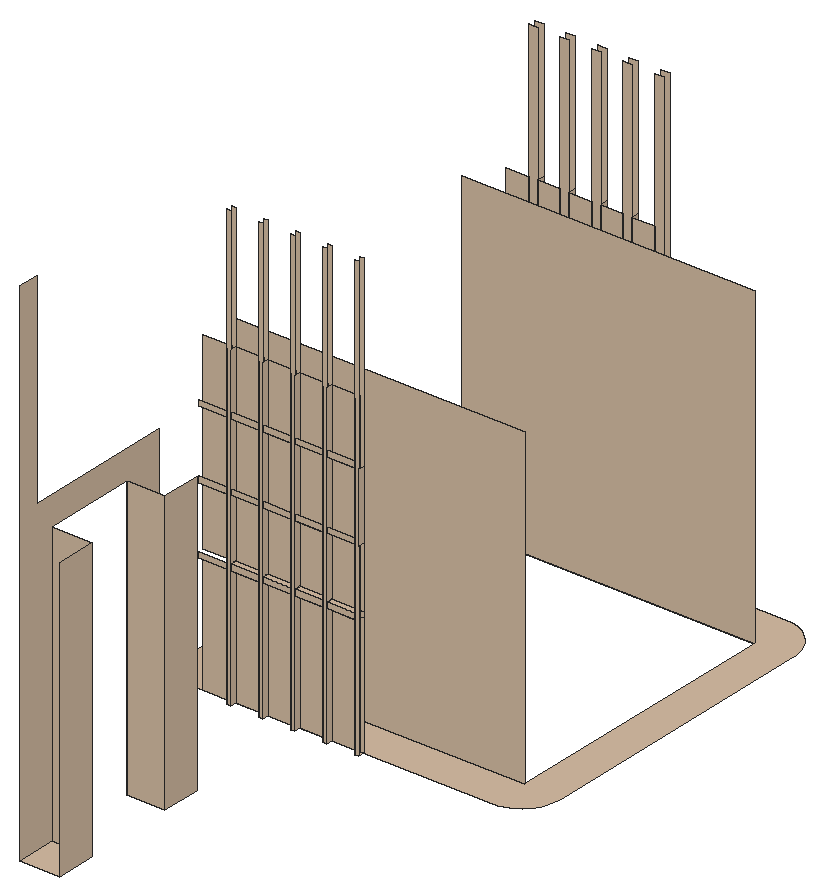
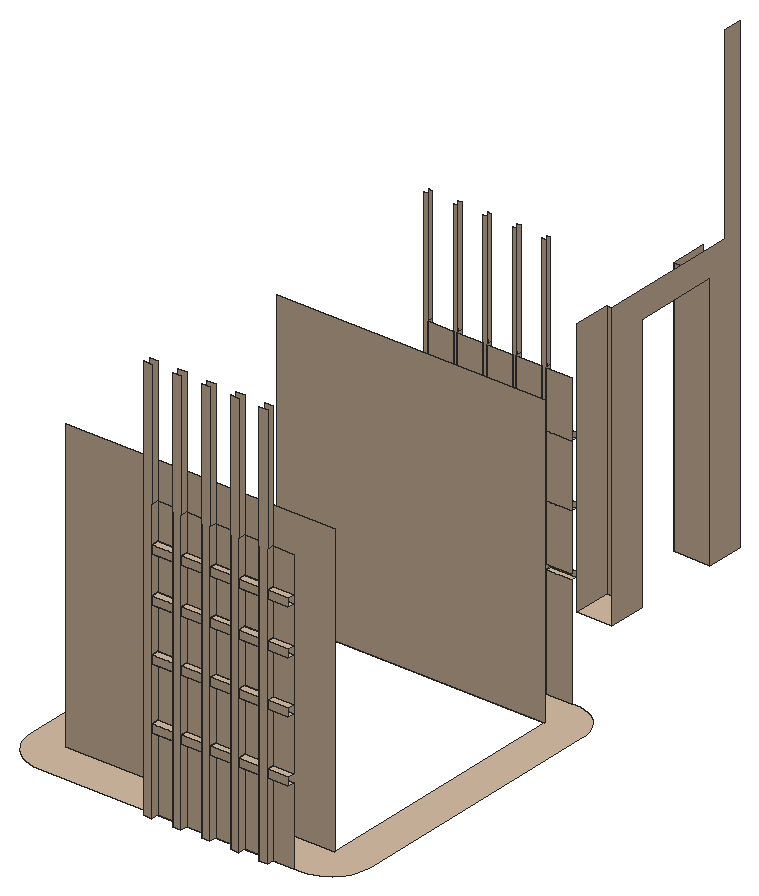
# SketchUp Ruby script. Lengths in inches.
U = 1.inch
M = Sketchup.active_model
def pt(a) = Geom::Point3d.new(a.map { |v| v * U })
def face(e, loops, mat)
  f = e.add_face(loops[0].map { |a| pt(a) })
  loops[1..].each { |l| e.add_face(l.map { |a| pt(a) }).erase! }
  f.material = f.back_material = mat if mat
  f
end
# faces: each face lists its corners as indices into pts; further lists are holes
def faces(e, pts, list, mat = nil) = list.each { |f| face(e, (f[0].is_a?(Array) ? f : [f]).map { |l| l.map { |i| pts[i] } }, mat) }
# xy, xz, yz: faces in a plane at the given z, y or x. An outline is a flat list of corners, or four numbers for a rectangle; further outlines are holes
def ring(l) = l.size == 4 ? [[l[0], l[1]], [l[2], l[1]], [l[2], l[3]], [l[0], l[3]]] : l.each_slice(2).to_a
def flat(e, list, mat, &to3) = list.each { |f| face(e, (f[0].is_a?(Array) ? f : [f]).map { |l| ring(l).map { |u, v| to3.(u, v) } }, mat) }
def xy(e, z, list, mat = nil) = flat(e, list, mat) { |x, y| [x, y, z] }
def xz(e, y, list, mat = nil) = flat(e, list, mat) { |x, z| [x, y, z] }
def yz(e, x, list, mat = nil) = flat(e, list, mat) { |y, z| [x, y, z] }
def lines(e, pts, list) = list.each { |a, b| e.add_line(pt(pts[a]), pt(pts[b])) }
# prism: a flat outline (further loops are holes) pulled along v
def prism(e, loops, v, mat = nil)
  f = face(e, loops, mat); d = Geom::Vector3d.new(v.map { |x| x * U })
  f.pushpull(f.normal.samedirection?(d) ? d.length : -d.length)
end
def box(e, o, s, mat = nil) = prism(e, [[o, [o[0] + s[0], o[1], o[2]], [o[0] + s[0], o[1] + s[1], o[2]], [o[0], o[1] + s[1], o[2]]]], [0, 0, s[2]], mat)
def at(x, y, z, deg = 0) = Geom::Transformation.translation(pt([x, y, z])) * Geom::Transformation.rotation(ORIGIN, Z_AXIS, deg.degrees)
def axes(o, x, y, z) = Geom::Transformation.new([*x, 0, *y, 0, *z, 0, *pt(o).to_a, 1])
def part(name) = M.definitions.add(name)
# library, detail: a bought-in or finely detailed component or shape, given as its bounding box
def library(name, o, s) = part(name).tap { |d| box(d.entities, o, s) }
def detail(e, o, s) = box(e.add_group.entities, o, s)
def put(e, d, t, mat = nil) = e.add_instance(d, t).tap { |i| i.material = mat if mat }
def group(e, t, mat = nil) = e.add_group.tap { |g| g.transformation = t; g.material = mat if mat }.entities
root = M.entities
M.materials.add("[Formica Laminate Light]").color = [213, 189, 164]
xy(root,0,[[297.89,97.95,301.53,101.59],[297.89,110.07,301.35,113.72],[295.1875,124.79,295.55,125.33],[298.11,124.79,298.47,125.33],[301.04,124.79,301.4,125.33],
  [303.96,124.79,304.32,125.33],[306.88,124.79,307.24,125.33],[[292.32,125.33,291.83,125.36,291.36,125.45,290.9,125.61,290.46,125.83,290.05,126.1,289.6875,126.42,289.37,126.78,289.1,127.1875,288.88,127.62,288.73,128.08,288.63,128.5625,288.6,129.05,288.6,155.08,288.63,155.58,288.72,156.07,288.88,156.55,289.09,157.01,289.36,157.43,289.68,157.82,290.04,158.16,290.45,158.46,290.89,158.7,291.35,158.89,291.84,159.02,292.34,159.08,318.9375,159.08,319.4,158.98,319.85,158.82,320.28,158.62,320.69,158.36,321.05,158.05,321.38,157.71,321.67,157.33,321.91,156.92,322.1,156.48,322.24,156.03,322.33,155.56,322.35,155.08,322.35,128.96,322.33,128.51,322.24,128.06,322.1,127.62,321.9,127.21,321.66,126.82,321.37,126.47,321.03,126.16,320.66,125.89,320.26,125.67,319.84,125.5,319.39,125.38,318.9375,125.33],[292.34,128.96,318.9375,155.08]],[295.2,159.08,296.03,159.77],[298.0625,159.08,298.89,159.77],
  [300.93,159.08,301.75,159.77],[303.79,159.08,304.62,159.77],[306.66,159.08,307.48,159.77]],"[Formica Laminate Light]")
xy(root,7.64,[[293.16,159.08,295.2,159.77],[296.03,159.08,298.0625,159.77],[298.89,159.08,300.93,159.77],[301.75,159.08,303.79,159.77],[304.62,159.08,306.66,159.77]],"[Formica Laminate Light]")
xy(root,8.44,[[293.16,159.08,295.2,159.77],[296.03,159.08,298.0625,159.77],[298.89,159.08,300.93,159.77],[301.75,159.08,303.79,159.77],[304.62,159.08,306.66,159.77]],"[Formica Laminate Light]")
xy(root,11.02,[[292.63,124.79,295.1875,125.33],[295.55,124.79,298.11,125.33],[298.47,124.79,301.04,125.33],[301.4,124.79,303.96,125.33],[304.32,124.79,306.88,125.33]],"[Formica Laminate Light]")
xy(root,11.55,[[295.55,124.79,298.11,125.33],[298.47,124.79,301.04,125.33],[301.4,124.79,303.96,125.33],[304.32,124.79,306.88,125.33]],"[Formica Laminate Light]")
xy(root,13.77,[[293.16,159.08,295.2,159.77],[296.03,159.08,298.0625,159.77],[298.89,159.08,300.93,159.77],[301.75,159.08,303.79,159.77],[304.62,159.08,306.66,159.77]],"[Formica Laminate Light]")
xy(root,14.57,[[293.16,159.08,295.2,159.77],[296.03,159.08,298.0625,159.77],[298.89,159.08,300.93,159.77],[301.75,159.08,303.79,159.77],[304.62,159.08,306.66,159.77]],"[Formica Laminate Light]")
xy(root,17.15,[[292.63,124.79,295.1875,125.33],[295.55,124.79,298.11,125.33],[298.47,124.79,301.04,125.33],[301.4,124.79,303.96,125.33],[304.32,124.79,306.88,125.33]],"[Formica Laminate Light]")
xy(root,19.01,[[293.16,159.08,295.2,159.77],[296.03,159.08,298.0625,159.77],[298.89,159.08,300.93,159.77],[301.75,159.08,303.79,159.77],[304.62,159.08,306.66,159.77]],"[Formica Laminate Light]")
xy(root,19.8125,[[293.16,159.08,295.2,159.77],[296.03,159.08,298.0625,159.77],[298.89,159.08,300.93,159.77],[301.75,159.08,303.79,159.77],[304.62,159.08,306.66,159.77]],"[Formica Laminate Light]")
xy(root,23.36,[[292.63,124.79,295.1875,125.33],[295.55,124.79,298.11,125.33],[298.47,124.79,301.04,125.33],[301.4,124.79,303.96,125.33],[304.32,124.79,306.88,125.33]],"[Formica Laminate Light]")
xy(root,23.54,[[293.16,159.08,295.2,159.77],[296.03,159.08,298.0625,159.77],[298.89,159.08,300.93,159.77],[301.75,159.08,303.79,159.77],[304.62,159.08,306.66,159.77]],"[Formica Laminate Light]")
xy(root,24.34,[[293.16,159.08,295.2,159.77],[296.03,159.08,298.0625,159.77],[298.89,159.08,300.93,159.77],[301.75,159.08,303.79,159.77],[304.62,159.08,306.66,159.77]],"[Formica Laminate Light]")
xz(root,101.59,[[297.89,0,301.53,25.5625]],"[Formica Laminate Light]")
xz(root,110.07,[[297.89,0,301.35,25.5625]],"[Formica Laminate Light]")
xz(root,124.79,[[295.1875,0,295.55,40.33],[298.11,0,298.47,40.33],[301.04,0,301.4,40.33],[303.96,0,304.32,40.33],[306.88,0,307.24,40.33],
  [292.63,11.02,295.1875,11.55],[295.55,11.02,298.11,11.55],[298.47,11.02,301.04,11.55],[301.4,11.02,303.96,11.55],[304.32,11.02,306.88,11.55],
  [292.63,17.15,295.1875,17.68],[295.55,17.15,298.11,17.68],[298.47,17.15,301.04,17.68],[301.4,17.15,303.96,17.68],[304.32,17.15,306.88,17.68],
  [292.63,23.36,295.1875,23.9],[295.55,23.36,298.11,23.9],[298.47,23.36,301.04,23.9],[301.4,23.36,303.96,23.9],[304.32,23.36,306.88,23.9]],"[Formica Laminate Light]")
xz(root,125.33,[[292.63,0,295.1875,11.02],[295.1875,0,295.55,11.02],[295.55,0,298.11,11.02],[298.11,0,298.47,11.02],[298.47,0,301.04,11.02],
  [301.04,0,301.4,11.02],[301.4,0,303.96,11.02],[303.96,0,304.32,11.02],[304.32,0,306.88,11.02],[306.88,0,307.24,11.02],
  [295.1875,11.02,295.55,11.55],[298.11,11.02,298.47,11.55],[301.04,11.02,301.4,11.55],[303.96,11.02,304.32,11.55],[306.88,11.02,307.24,11.55],
  [292.63,11.55,295.1875,17.15],[295.1875,11.55,295.55,40.33],[295.55,11.55,298.11,17.15],[298.11,11.55,298.47,40.33],[298.47,11.55,301.04,17.15],
  [301.04,11.55,301.4,40.33],[301.4,11.55,303.96,17.15],[303.96,11.55,304.32,40.33],[304.32,11.55,306.88,17.15],[306.88,11.55,307.24,40.33],
  [292.63,17.15,295.1875,23.36],[295.55,17.15,298.11,23.36],[298.47,17.15,301.04,23.36],[301.4,17.15,303.96,23.36],[304.32,17.15,306.88,23.36],
  [292.63,23.36,295.1875,28.96],[295.55,23.36,298.11,28.96],[298.47,23.36,301.04,28.96],[301.4,23.36,303.96,28.96],[304.32,23.36,306.88,28.96]],"[Formica Laminate Light]")
xz(root,128.96,[[292.34,0,318.9375,28.69]],"[Formica Laminate Light]")
xz(root,155.08,[[292.34,0,318.9375,28.69]],"[Formica Laminate Light]")
xz(root,159.08,[[293.16,0,295.2,7.64],[295.2,0,296.03,40.33],[296.03,0,298.0625,7.64],[298.0625,0,298.89,40.33],[298.89,0,300.93,7.64],
  [300.93,0,301.75,40.33],[301.75,0,303.79,7.64],[303.79,0,304.62,40.33],[304.62,0,306.66,7.64],[306.66,0,307.48,40.33],
  [293.16,8.44,295.2,13.77],[296.03,8.44,298.0625,13.77],[298.89,8.44,300.93,13.77],[301.75,8.44,303.79,13.77],[304.62,8.44,306.66,13.77],
  [293.16,13.77,295.2,14.57],[296.03,13.77,298.0625,14.57],[298.89,13.77,300.93,14.57],[301.75,13.77,303.79,14.57],[304.62,13.77,306.66,14.57],
  [293.16,14.57,295.2,19.01],[296.03,14.57,298.0625,19.01],[298.89,14.57,300.93,19.01],[301.75,14.57,303.79,19.01],[304.62,14.57,306.66,19.01],
  [293.16,19.01,295.2,19.8125],[296.03,19.01,298.0625,19.8125],[298.89,19.01,300.93,19.8125],[301.75,19.01,303.79,19.8125],[304.62,19.01,306.66,19.8125],
  [293.16,19.8125,295.2,23.54],[296.03,19.8125,298.0625,23.54],[298.89,19.8125,300.93,23.54],[301.75,19.8125,303.79,23.54],[304.62,19.8125,306.66,23.54],
  [293.16,23.54,295.2,24.34],[296.03,23.54,298.0625,24.34],[298.89,23.54,300.93,24.34],[301.75,23.54,303.79,24.34],[304.62,23.54,306.66,24.34],
  [293.16,24.34,295.2,27.9],[296.03,24.34,298.0625,27.9],[298.89,24.34,300.93,27.9],[301.75,24.34,303.79,27.9],[304.62,24.34,306.66,27.9]],"[Formica Laminate Light]")
xz(root,159.77,[[295.2,0,296.03,40.33],[298.0625,0,298.89,40.33],[300.93,0,301.75,40.33],[303.79,0,304.62,40.33],[306.66,0,307.48,40.33],
  [293.16,7.64,295.2,8.44],[296.03,7.64,298.0625,8.44],[298.89,7.64,300.93,8.44],[301.75,7.64,303.79,8.44],[304.62,7.64,306.66,8.44],
  [293.16,13.77,295.2,14.57],[296.03,13.77,298.0625,14.57],[298.89,13.77,300.93,14.57],[301.75,13.77,303.79,14.57],[304.62,13.77,306.66,14.57],
  [293.16,19.01,295.2,19.8125],[296.03,19.01,298.0625,19.8125],[298.89,19.01,300.93,19.8125],[301.75,19.01,303.79,19.8125],[304.62,19.01,306.66,19.8125],
  [293.16,23.54,295.2,24.34],[296.03,23.54,298.0625,24.34],[298.89,23.54,300.93,24.34],[301.75,23.54,303.79,24.34],[304.62,23.54,306.66,24.34]],"[Formica Laminate Light]")
yz(root,295.1875,[[124.79,0,125.33,11.02],[124.79,11.02,125.33,11.55],[124.79,11.55,125.33,17.15],[124.79,17.15,125.33,23.36],[124.79,23.36,125.33,28.96]],"[Formica Laminate Light]")
yz(root,295.2,[[159.08,0,159.77,7.64],[159.08,7.64,159.77,8.44],[159.08,8.44,159.77,13.77],[159.08,13.77,159.77,14.57],[159.08,14.57,159.77,19.01],
  [159.08,19.01,159.77,19.8125],[159.08,19.8125,159.77,23.54],[159.08,23.54,159.77,24.34],[159.08,24.34,159.77,27.9]],"[Formica Laminate Light]")
yz(root,295.55,[[124.79,0,125.33,11.02],[124.79,11.02,125.33,11.55],[124.79,11.55,125.33,17.15],[124.79,17.15,125.33,23.36],[124.79,23.36,125.33,28.96]],"[Formica Laminate Light]")
yz(root,296.03,[[159.08,0,159.77,7.64],[159.08,7.64,159.77,8.44],[159.08,8.44,159.77,13.77],[159.08,13.77,159.77,14.57],[159.08,14.57,159.77,19.01],
  [159.08,19.01,159.77,19.8125],[159.08,19.8125,159.77,23.54],[159.08,23.54,159.77,24.34],[159.08,24.34,159.77,27.9]],"[Formica Laminate Light]")
yz(root,297.89,[[97.95,0,97.95,46.82,99.82,46.82,99.82,28.25,113.72,28.25,113.72,0,110.07,0,110.07,25.5625,101.59,25.5625,101.59,0]],"[Formica Laminate Light]")
yz(root,298.0625,[[159.08,0,159.77,7.64],[159.08,7.64,159.77,8.44],[159.08,8.44,159.77,13.77],[159.08,13.77,159.77,14.57],[159.08,14.57,159.77,19.01],
  [159.08,19.01,159.77,19.8125],[159.08,19.8125,159.77,23.54],[159.08,23.54,159.77,24.34],[159.08,24.34,159.77,27.9]],"[Formica Laminate Light]")
yz(root,298.11,[[124.79,0,125.33,11.02],[124.79,11.02,125.33,11.55],[124.79,11.55,125.33,17.15],[124.79,17.15,125.33,23.36],[124.79,23.36,125.33,28.96]],"[Formica Laminate Light]")
yz(root,298.47,[[124.79,0,125.33,11.02],[124.79,11.02,125.33,11.55],[124.79,11.55,125.33,17.15],[124.79,17.15,125.33,23.36],[124.79,23.36,125.33,28.96]],"[Formica Laminate Light]")
yz(root,298.89,[[159.08,0,159.77,7.64],[159.08,7.64,159.77,8.44],[159.08,8.44,159.77,13.77],[159.08,13.77,159.77,14.57],[159.08,14.57,159.77,19.01],
  [159.08,19.01,159.77,19.8125],[159.08,19.8125,159.77,23.54],[159.08,23.54,159.77,24.34],[159.08,24.34,159.77,27.9]],"[Formica Laminate Light]")
yz(root,300.93,[[159.08,0,159.77,7.64],[159.08,7.64,159.77,8.44],[159.08,8.44,159.77,13.77],[159.08,13.77,159.77,14.57],[159.08,14.57,159.77,19.01],
  [159.08,19.01,159.77,19.8125],[159.08,19.8125,159.77,23.54],[159.08,23.54,159.77,24.34],[159.08,24.34,159.77,27.9]],"[Formica Laminate Light]")
yz(root,301.04,[[124.79,0,125.33,11.02],[124.79,11.02,125.33,11.55],[124.79,11.55,125.33,17.15],[124.79,17.15,125.33,23.36],[124.79,23.36,125.33,28.96]],"[Formica Laminate Light]")
yz(root,301.35,[[110.07,0,113.72,25.5625]],"[Formica Laminate Light]")
yz(root,301.4,[[124.79,0,125.33,11.02],[124.79,11.02,125.33,11.55],[124.79,11.55,125.33,17.15],[124.79,17.15,125.33,23.36],[124.79,23.36,125.33,28.96]],"[Formica Laminate Light]")
yz(root,301.53,[[97.95,0,101.59,25.5625]],"[Formica Laminate Light]")
yz(root,301.75,[[159.08,0,159.77,7.64],[159.08,7.64,159.77,8.44],[159.08,8.44,159.77,13.77],[159.08,13.77,159.77,14.57],[159.08,14.57,159.77,19.01],
  [159.08,19.01,159.77,19.8125],[159.08,19.8125,159.77,23.54],[159.08,23.54,159.77,24.34],[159.08,24.34,159.77,27.9]],"[Formica Laminate Light]")
yz(root,303.79,[[159.08,0,159.77,7.64],[159.08,7.64,159.77,8.44],[159.08,8.44,159.77,13.77],[159.08,13.77,159.77,14.57],[159.08,14.57,159.77,19.01],
  [159.08,19.01,159.77,19.8125],[159.08,19.8125,159.77,23.54],[159.08,23.54,159.77,24.34],[159.08,24.34,159.77,27.9]],"[Formica Laminate Light]")
yz(root,303.96,[[124.79,0,125.33,11.02],[124.79,11.02,125.33,11.55],[124.79,11.55,125.33,17.15],[124.79,17.15,125.33,23.36],[124.79,23.36,125.33,28.96]],"[Formica Laminate Light]")
yz(root,304.32,[[124.79,0,125.33,11.02],[124.79,11.02,125.33,11.55],[124.79,11.55,125.33,17.15],[124.79,17.15,125.33,23.36],[124.79,23.36,125.33,28.96]],"[Formica Laminate Light]")
yz(root,304.62,[[159.08,0,159.77,7.64],[159.08,7.64,159.77,8.44],[159.08,8.44,159.77,13.77],[159.08,13.77,159.77,14.57],[159.08,14.57,159.77,19.01],
  [159.08,19.01,159.77,19.8125],[159.08,19.8125,159.77,23.54],[159.08,23.54,159.77,24.34],[159.08,24.34,159.77,27.9]],"[Formica Laminate Light]")
yz(root,306.66,[[159.08,0,159.77,7.64],[159.08,7.64,159.77,8.44],[159.08,8.44,159.77,13.77],[159.08,13.77,159.77,14.57],[159.08,14.57,159.77,19.01],
  [159.08,19.01,159.77,19.8125],[159.08,19.8125,159.77,23.54],[159.08,23.54,159.77,24.34],[159.08,24.34,159.77,27.9]],"[Formica Laminate Light]")
yz(root,306.88,[[124.79,0,125.33,11.02],[124.79,11.02,125.33,11.55],[124.79,11.55,125.33,17.15],[124.79,17.15,125.33,23.36],[124.79,23.36,125.33,28.96]],"[Formica Laminate Light]")
yz(root,307.24,[[124.79,17.15,125.33,23.36]],"[Formica Laminate Light]")
